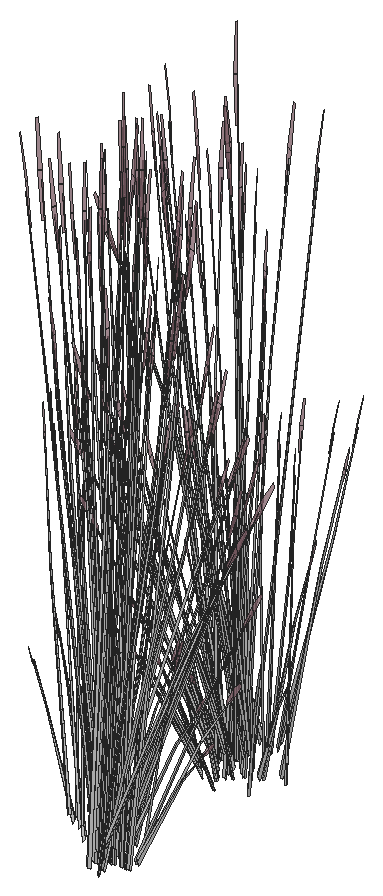
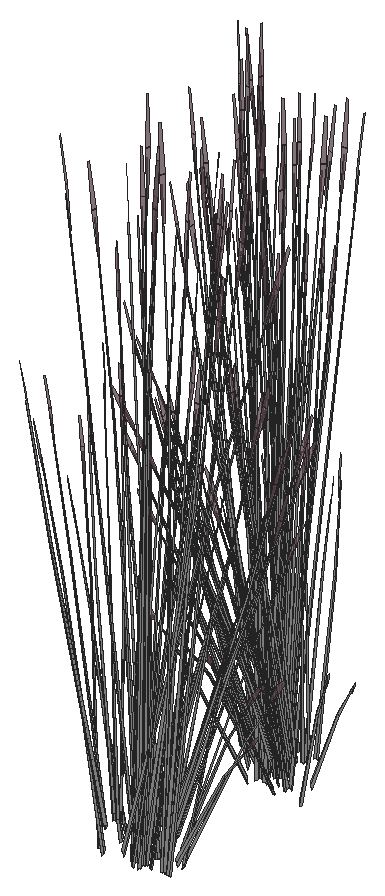
# SketchUp Ruby script. Lengths in inches.
U = 1.inch
M = Sketchup.active_model
def pt(a) = Geom::Point3d.new(a.map { |v| v * U })
def face(e, loops, mat)
  f = e.add_face(loops[0].map { |a| pt(a) })
  loops[1..].each { |l| e.add_face(l.map { |a| pt(a) }).erase! }
  f.material = f.back_material = mat if mat
  f
end
# faces: each face lists its corners as indices into pts; further lists are holes
def faces(e, pts, list, mat = nil) = list.each { |f| face(e, (f[0].is_a?(Array) ? f : [f]).map { |l| l.map { |i| pts[i] } }, mat) }
# xy, xz, yz: faces in a plane at the given z, y or x. An outline is a flat list of corners, or four numbers for a rectangle; further outlines are holes
def ring(l) = l.size == 4 ? [[l[0], l[1]], [l[2], l[1]], [l[2], l[3]], [l[0], l[3]]] : l.each_slice(2).to_a
def flat(e, list, mat, &to3) = list.each { |f| face(e, (f[0].is_a?(Array) ? f : [f]).map { |l| ring(l).map { |u, v| to3.(u, v) } }, mat) }
def xy(e, z, list, mat = nil) = flat(e, list, mat) { |x, y| [x, y, z] }
def xz(e, y, list, mat = nil) = flat(e, list, mat) { |x, z| [x, y, z] }
def yz(e, x, list, mat = nil) = flat(e, list, mat) { |y, z| [x, y, z] }
def lines(e, pts, list) = list.each { |a, b| e.add_line(pt(pts[a]), pt(pts[b])) }
# prism: a flat outline (further loops are holes) pulled along v
def prism(e, loops, v, mat = nil)
  f = face(e, loops, mat); d = Geom::Vector3d.new(v.map { |x| x * U })
  f.pushpull(f.normal.samedirection?(d) ? d.length : -d.length)
end
def box(e, o, s, mat = nil) = prism(e, [[o, [o[0] + s[0], o[1], o[2]], [o[0] + s[0], o[1] + s[1], o[2]], [o[0], o[1] + s[1], o[2]]]], [0, 0, s[2]], mat)
def at(x, y, z, deg = 0) = Geom::Transformation.translation(pt([x, y, z])) * Geom::Transformation.rotation(ORIGIN, Z_AXIS, deg.degrees)
def axes(o, x, y, z) = Geom::Transformation.new([*x, 0, *y, 0, *z, 0, *pt(o).to_a, 1])
def part(name) = M.definitions.add(name)
# library, detail: a bought-in or finely detailed component or shape, given as its bounding box
def library(name, o, s) = part(name).tap { |d| box(d.entities, o, s) }
def detail(e, o, s) = box(e.add_group.entities, o, s)
def put(e, d, t, mat = nil) = e.add_instance(d, t).tap { |i| i.material = mat if mat }
def group(e, t, mat = nil) = e.add_group.tap { |g| g.transformation = t; g.material = mat if mat }.entities
root = M.entities
M.materials.add("LightPink_Translucent").color = [144, 107, 117]
M.materials["LightPink_Translucent"].alpha = 0.75
M.materials.add("[_0053_Ivory_]").color = [200, 200, 200]
c1 = part("blade")
p = [[2.15,0.21,22],[0,0.17,0],[0.09,0.45,0],[2.18,0.31,22],[2.29,0.31,22],[0.38,0.45,0],
  [2.48,0.24,33],[2.49,0.24,33],[2.48,0.22,33]]
faces(c1.entities,p,[[0,1,2,3],[4,5,2,3],[6,3,4,7],[8,0,3,6]])
c2 = part("seeds")
p = [[0.3,-0.1,1.38],[-0.01,-0.03,1.59],[-0.01,-0.03,0.03],[0.14,-0.07,-0.07],[0.29,-0.03,3],[0.15,0.01,3.11]]
faces(c2.entities,p,[[0,1,2,3],[1,0,4,5]],"LightPink_Translucent")
c3 = part("blade with seeds")
put(c3.entities,c1,at(0,0,0))
put(c3.entities,c2,axes([2.4,0.25,30.99],[1.5799,-0.05474,1.17369],[-0.12525,1.92788,0.29478],[-0.07173,-0.02425,1.56792]))
put(root,c3,axes([645.01,152.18,129.13],[-0.65264,0.16691,0.17642],[-0.16115,-0.62115,0.35086],[0.05821,0.0905,1.60407]),"[_0053_Ivory_]")
put(root,c3,axes([645.42,153.49,130.53],[-0.25192,0.01424,1.71376],[0.16712,-0.61729,0.13857],[0.35901,0.03818,0.73262]),"[_0053_Ivory_]")
put(root,c3,axes([645.74,152.15,128.68],[0.14267,0.54795,-0.30978],[-0.56663,0.1556,0.30978],[0.11423,0.06319,1.38974]),"[_0053_Ivory_]")
put(root,c3,axes([644.6,153.375,129.03],[-0.76764,-0.13249,0.49198],[0.15622,-0.74829,0.19306],[0.11218,0.07226,1.70813]),"[_0053_Ivory_]")
put(root,c3,axes([643.99,155.22,128.86],[-0.19817,-0.54216,0],[0.56587,-0.18986,0],[0,0,1.54371]),"[_0053_Ivory_]")
put(root,c3,axes([643.61,154.71,129.27],[-0.11717,0.56122,0.1448],[-0.57245,-0.09742,-0.41347],[-0.10418,-0.05763,1.26744]),"[_0053_Ivory_]")
put(root,c3,axes([644.73,155.14,128.84],[0.63764,-0.21337,-0.19198],[0.22406,0.61462,0.00008],[0.07038,-0.02358,1.73897]),"[_0053_Ivory_]")
put(root,c3,axes([644.95,155.4,129.13],[0.17545,-0.62497,0.17642],[0.64204,0.17686,0.35086],[-0.11091,0.00304,1.60407]),"[_0053_Ivory_]")
put(root,c3,axes([644.81,153.98,128.87],[0.42396,0.40619,0],[-0.42396,0.40619,0],[0,0,1.69266]),"[_0053_Ivory_]")
put(root,c3,axes([645.95,153.81,129.13],[-0.47719,-0.45806,0.17642],[0.48088,-0.44429,0.35086],[-0.0527,0.09355,1.60407]),"[_0053_Ivory_]")
put(root,c3,axes([645.07,153.12,128.71],[0.63179,0.1031,-0.62353],[-0.13332,0.63596,-0.16365],[0.18854,0.07706,1.37633]),"[_0053_Ivory_]")
put(root,c3,axes([647.86,154.23,129.42],[-0.37526,0.10382,1.1486],[0.17664,-0.42906,0.84392],[0.19907,0.02936,0.25299]),"[_0053_Ivory_]")
put(root,c3,axes([643.85,155.47,128.85],[-0.61229,-0.28233,0],[0.29468,-0.58663,0],[0,0,1.62707]),"[_0053_Ivory_]")
put(root,c3,axes([644.36,154.71,129.12],[-0.59306,-0.50614,-0.25192],[0.49904,-0.56836,0.5513],[-0.1597,0.05921,1.68216]),"[_0053_Ivory_]")
put(root,c3,axes([642.8,155.68,129.13],[0.56842,0.31443,0.49651],[-0.33976,0.56381,0],[-0.12946,-0.07161,1.57504]),"[_0053_Ivory_]")
put(root,c3,axes([644.8,153.51,129.37],[0.29468,-0.56664,0.44739],[0.61229,0.27271,-0.21531],[0,0.13062,1.43643]),"[_0053_Ivory_]")
put(root,c3,axes([644.6875,153.83,128.95],[0,0.72727,-0.05637],[-0.75945,0,0],[0,0.02286,1.79368]),"[_0053_Ivory_]")
put(root,c3,axes([644.74,153.32,128.86],[0.36485,0.52782,-0.44739],[-0.55265,0.37168,0.21531],[0.11807,0.06531,1.43643]),"[_0053_Ivory_]")
put(root,c3,axes([647.21,155.55,130.58],[-0.11624,-0.52862,-0.03492],[0.54943,-0.12153,-0.15832],[0.11473,0.03351,0.52218]),"[_0053_Ivory_]")
put(root,c3,axes([642.47,156.01,129.03],[-0.37973,0.63014,0],[-0.6353,-0.35142,-0.51607],[-0.14469,-0.08004,1.63711]),"[_0053_Ivory_]")
put(root,c3,axes([646.35,153.82,129.13],[0,-0.62885,0.49651],[0.67951,0,0],[0,0.14322,1.57504]),"[_0053_Ivory_]")
put(root,c3,axes([644.65,154.29,129.37],[0.65953,-0.03882,0.44739],[0.05964,0.64439,-0.21531],[-0.11807,0.06531,1.43643]),"[_0053_Ivory_]")
put(root,c3,axes([645.06,153.64,129.27],[0.56587,-0.18339,0.1448],[0.19817,0.52368,-0.41347],[0,0.11525,1.26744]),"[_0053_Ivory_]")
put(root,c3,axes([644.06,154.61,128.86],[-0.65953,0.03882,-0.44739],[-0.05964,-0.64439,0.21531],[-0.11807,0.06531,1.43643]),"[_0053_Ivory_]")
put(root,c3,axes([647.16,154.91,129.24],[-0.14627,-0.15466,1.43002],[0.19032,-0.51164,-0.30754],[0.29594,0.06931,0.61141]),"[_0053_Ivory_]")
put(root,c3,axes([644.55,155.48,128.86],[0.61229,0.28233,0],[-0.29468,0.58663,0],[0,0,1.74954]),"[_0053_Ivory_]")
put(root,c3,axes([644.79,156.1,128.85],[-0.37499,-0.63235,-0.05142],[0.6353,-0.35142,0.51607],[-0.15655,0.0602,1.6363]),"[_0053_Ivory_]")
put(root,c3,axes([644.66,154.57,129.27],[0.44871,0.37783,0.1448],[-0.37428,0.42627,-0.41347],[-0.10418,0.05763,1.26744]),"[_0053_Ivory_]")
put(root,c3,axes([645.82,155.23,131.63],[0.60713,0.01514,-0.71045],[-0.04078,0.63759,0.08574],[0.25721,0.06729,1.00501]),"[_0053_Ivory_]")
put(root,c3,axes([645.13,155.74,129.13],[0.56842,-0.31443,0.49651],[0.33976,0.56381,0],[-0.12946,0.07161,1.57504]),"[_0053_Ivory_]")
put(root,c3,axes([644.32,155.24,128.94],[0.26406,0.72244,-0.06012],[-0.7545,0.25315,0],[0.00922,0.02523,1.72173]),"[_0053_Ivory_]")
put(root,c3,axes([644.62,156.02,128.68],[-0.56663,-0.1556,-0.30978],[0.14267,-0.54795,0.30978],[-0.11423,0.06319,1.38974]),"[_0053_Ivory_]")
put(root,c3,axes([646.81,153.93,129.03],[0.75945,0,0],[0,0.70283,-0.51607],[0,0.16007,1.63711]),"[_0053_Ivory_]")
put(root,c3,axes([646.51,154.29,128.85],[-0.75908,-0.00503,-0.04976],[0,-0.70283,0.49943],[-0.02386,0.16,1.58352]),"[_0053_Ivory_]")
put(root,c3,axes([644.86,153.68,129.32],[0.68399,0.30005,-0.29095],[-0.32934,0.63331,-0.50002],[0.0215,0.15549,1.59708]),"[_0053_Ivory_]")
put(root,c3,axes([640.09,156.01,129.42],[0.25312,-0.28501,1.1486],[0.09988,0.45119,0.84392],[-0.18292,0.08079,0.25299]),"[_0053_Ivory_]")
put(root,c3,axes([646.18,155.49,131.18],[0.34557,0.39372,-0.35414],[-0.39459,0.37271,0.4572],[0.20048,0.05671,0.87481]),"[_0053_Ivory_]")
put(root,c3,axes([646.35,154.39,128.68],[-0.42396,0.39235,-0.30978],[-0.42396,-0.39235,0.30978],[0,0.12637,1.38974]),"[_0053_Ivory_]")
put(root,c3,axes([644.52,154.43,129.32],[0.07077,0.71755,-0.29095],[-0.73712,0.04339,-0.50002],[-0.1298,0.09558,1.59708]),"[_0053_Ivory_]")
put(root,c3,axes([644.79,154.15,128.86],[-0.29468,0.56664,-0.44739],[-0.61229,-0.27271,0.21531],[0,0.13062,1.43643]),"[_0053_Ivory_]")
put(root,c3,axes([641.04,154.78,131.18],[-0.52868,0.08987,-0.35414],[-0.1396,-0.51376,0.4572],[-0.1515,0.13799,0.87481]),"[_0053_Ivory_]")
put(root,c3,axes([644.08,154.98,128.71],[-0.40909,0.47266,-0.62353],[-0.50819,-0.4286,-0.16365],[-0.16393,0.11791,1.37633]),"[_0053_Ivory_]")
put(root,c3,axes([644.81,155.78,128.98],[0.76036,0.2044,0.30756],[-0.19023,0.7306,-0.36492],[-0.12585,0.09144,1.64885]),"[_0053_Ivory_]")
put(root,c3,axes([644.75,156.27,128.67],[-0.56842,0.31443,-0.49651],[-0.33976,-0.56381,0],[-0.12946,0.07161,1.57504]),"[_0053_Ivory_]")
put(root,c3,axes([646.64,154.41,128.67],[0,0.62885,-0.49651],[-0.67951,0,0],[0,0.14322,1.57504]),"[_0053_Ivory_]")
put(root,c3,axes([644.94,154.48,130.53],[-0.2256,-0.10835,1.71376],[0.46687,-0.45453,0.13857],[0.29098,0.20505,0.73262]),"[_0053_Ivory_]")
put(root,c3,axes([645.78,155.71,129.42],[-0.34197,-0.18082,1.1486],[0.44156,-0.18372,0.84392],[0.1191,0.15563,0.25299]),"[_0053_Ivory_]")
put(root,c3,axes([641.96,154.28,130.53],[0.1517,-0.19322,1.71376],[0.38303,0.52154,0.13857],[-0.26271,0.23751,0.73262]),"[_0053_Ivory_]")
put(root,c3,axes([641.48,154.84,131.33],[0.15602,0.5742,-0.51099],[-0.59087,0.10045,-0.3958],[-0.16933,0.15423,0.97773]),"[_0053_Ivory_]")
put(root,c3,axes([645.27,156.17,129.03],[0.37973,0.63014,0],[-0.6353,0.35142,-0.51607],[-0.14469,0.08004,1.63711]),"[_0053_Ivory_]")
put(root,c3,axes([645.87,156.38,128.15],[0.04425,-0.09079,1.76342],[0.55709,-0.26738,-0.26939],[0.16889,0.13839,0.30037]),"[_0053_Ivory_]")
put(root,c3,axes([644.94,153.68,129.5],[-0.01659,-0.59209,1.41272],[0.75089,0.15348,0.59816],[-0.1776,0.32398,1.3335]),"[_0053_Ivory_]")
put(root,c3,axes([645.14,154.32,128.75],[0.2227,0.57576,-0.69212],[-0.64151,0.20736,-0.18165],[0.02462,0.19497,1.52773]),"[_0053_Ivory_]")
put(root,c3,axes([640.76,156.31,128.15],[0.08147,0.06283,1.76342],[0.13814,0.58211,-0.26939],[-0.18056,0.12413,0.30037]),"[_0053_Ivory_]")
put(root,c3,axes([645,155.96,131.33],[0.59932,-0.14948,-0.51099],[0.10484,0.56611,-0.3958],[0.16097,0.16223,0.97773]),"[_0053_Ivory_]")
put(root,c3,axes([645.83,156.54,129.32],[-0.38947,-0.01972,1.0506],[0.25721,-0.41888,0.58006],[0.15386,0.14882,0.8241]),"[_0053_Ivory_]")
put(root,c3,axes([641.84,154.75,130.53],[0.11309,-0.21615,1.71376],[0.47441,0.44731,0.13857],[-0.21402,0.27879,0.73262]),"[_0053_Ivory_]")
put(root,c3,axes([644.56,155.52,129.24],[0.01072,-0.20846,1.43002],[0.51218,-0.23285,-0.30754],[0.15811,0.2495,0.61141]),"[_0053_Ivory_]")
put(root,c3,axes([641.97,155.97,131.18],[-0.41095,0.33109,-0.35414],[-0.38901,-0.37805,0.4572],[-0.05919,0.19208,0.87481]),"[_0053_Ivory_]")
put(root,c3,axes([642.24,157.26,129.42],[-0.01572,-0.37392,1.1486],[0.39276,0.26669,0.84392],[-0.07724,0.17822,0.25299]),"[_0053_Ivory_]")
put(root,c3,axes([643.27,156.36,128.15],[0.09829,-0.03422,1.76342],[0.59126,0.18834,-0.26939],[0.01729,0.21228,0.30037]),"[_0053_Ivory_]")
put(root,c3,axes([642.38,155.82,131.66],[0.43478,0.42253,-0.5672],[-0.45929,0.37004,-0.43934],[-0.06615,0.21468,1.08528]),"[_0053_Ivory_]")
put(root,c3,axes([641.91,156.45,129.48],[0.55175,-0.11136,0.06507],[0.12684,0.44864,-0.86304],[-0.03498,0.22711,0.7736]),"[_0053_Ivory_]")
put(root,c3,axes([643.67,156.22,131.33],[0.59704,0.15764,-0.51099],[-0.20464,0.54049,-0.3958],[0.05475,0.21761,0.97773]),"[_0053_Ivory_]")
put(root,c3,axes([644.01,155.11,130.53],[-0.13883,-0.2019,1.71376],[0.64153,-0.16998,0.13857],[0.14499,0.31697,0.73262]),"[_0053_Ivory_]")
put(root,c3,axes([643.4,156.56,131.18],[-0.1831,0.48359,-0.35414],[-0.53419,-0.14105,0.4572],[0.04898,0.1947,0.87481]),"[_0053_Ivory_]")
put(root,c3,axes([642.25,155.62,131.99],[-0.0158,0.58168,-0.7886],[-0.66548,-0.03907,0.09517],[-0.07023,0.24643,1.11556]),"[_0053_Ivory_]")
put(root,c3,axes([642.88,155.21,130.53],[-0.01487,-0.24136,1.71376],[0.64429,0.16012,0.13857],[-0.03985,0.34396,0.73262]),"[_0053_Ivory_]")
put(root,c3,axes([643.46,156.12,131.63],[0.28988,0.51132,-0.71045],[-0.59671,0.28496,0.08574],[0.06778,0.24706,1.00501]),"[_0053_Ivory_]")
put(root,c3,axes([641.78,156.93,129.24],[0.19166,-0.0992,1.43002],[0.4732,0.29912,-0.30754],[-0.14084,0.25882,0.61141]),"[_0053_Ivory_]")
put(root,c3,axes([642.03,156.44,130.02],[0.01334,-0.32463,1.54345],[0.60018,0.17147,0.21329],[-0.052,0.34598,0.72882]),"[_0053_Ivory_]")
put(root,c3,axes([642.49,169.64,130.53],[0.13883,0.2019,1.71376],[-0.64153,0.16998,0.13857],[-0.14499,-0.31697,0.73262]),"[_0053_Ivory_]")
put(root,c3,axes([644.98,169.35,129.24],[-0.17264,0.12729,1.43002],[-0.51703,-0.22279,-0.30754],[0.09584,-0.27707,0.61141]),"[_0053_Ivory_]")
put(root,c3,axes([644.2,169.79,131.63],[-0.28988,-0.51132,-0.71045],[0.59671,-0.28496,0.08574],[-0.06778,-0.24706,1.00501]),"[_0053_Ivory_]")
put(root,c3,axes([642.3125,169.11,129.24],[-0.03678,0.20572,1.43002],[-0.53767,0.17221,-0.30754],[-0.12568,-0.26589,0.61141]),"[_0053_Ivory_]")
put(root,c3,axes([643.7,168.66,128.15],[-0.10187,0.02266,1.76342],[-0.56336,-0.25503,-0.26939],[0.00945,-0.21273,0.30037]),"[_0053_Ivory_]")
put(root,c3,axes([645.4,170.29,131.63],[0.0158,-0.58168,-0.71045],[0.66548,0.03907,0.08574],[0.07023,-0.24643,1.00501]),"[_0053_Ivory_]")
put(root,c3,axes([644.25,169.36,131.18],[0.1831,-0.48359,-0.35414],[0.53419,0.14105,0.4572],[-0.04898,-0.1947,0.87481]),"[_0053_Ivory_]")
put(root,c3,axes([644.65,170,130.53],[-0.11309,0.21615,1.71376],[-0.47441,-0.44731,0.13857],[0.21402,-0.27879,0.73262]),"[_0053_Ivory_]")
put(root,c3,axes([643.98,169.6875,131.33],[-0.59704,-0.15764,-0.51099],[0.20464,-0.54049,-0.3958],[-0.05475,-0.21761,0.97773]),"[_0053_Ivory_]")
put(root,c3,axes([644.35,168.33,129.42],[0.07791,0.3667,1.1486],[-0.43222,-0.2031,0.84392],[0.04651,-0.18776,0.25299]),"[_0053_Ivory_]")
put(root,c3,axes([645.27,170.1,131.33],[-0.43478,-0.42253,-0.51099],[0.45929,-0.37004,-0.3958],[0.06615,-0.21468,0.97773]),"[_0053_Ivory_]")
put(root,c3,axes([645.68,169.94,131.18],[0.41095,-0.33109,-0.35414],[0.38901,0.37805,0.4572],[0.05919,-0.19208,0.87481]),"[_0053_Ivory_]")
put(root,c3,axes([642.125,168.77,129.42],[0.31682,0.21887,1.1486],[-0.4614,0.13157,0.84392],[-0.09872,-0.16821,0.25299]),"[_0053_Ivory_]")
put(root,c3,axes([642.89,169.94,131.63],[-0.51789,-0.30395,-0.71045],[0.36805,-0.53263,0.08574],[-0.18764,-0.18149,1.00501]),"[_0053_Ivory_]")
put(root,c3,axes([642.71,169.53,131.18],[-0.0938,-0.50652,-0.35414],[0.53623,-0.13375,0.4572],[-0.14403,-0.14515,0.87481]),"[_0053_Ivory_]")
put(root,c3,axes([641.875,169.43,128.15],[-0.05883,0.08284,1.76342],[-0.59454,0.17861,-0.26939],[-0.14363,-0.16248,0.30037]),"[_0053_Ivory_]")
put(root,c3,axes([642.86,171.71,128.75],[-0.24943,-0.64486,-0.69835],[0.71849,-0.23224,-0.18329],[-0.02757,-0.21836,1.54149]),"[_0053_Ivory_]")
put(root,c3,axes([646.19,169.74,128.15],[-0.0909,-0.04954,1.76342],[-0.2335,-0.55347,-0.26939],[0.15752,-0.1502,0.30037]),"[_0053_Ivory_]")
put(root,c3,axes([642.65,169.95,131.33],[-0.59932,0.14948,-0.51099],[-0.10484,-0.56611,-0.3958],[-0.16097,-0.16223,0.97773]),"[_0053_Ivory_]")
put(root,c3,axes([646.1875,171.3,131.63],[0.31725,-0.49618,-0.71045],[0.55593,0.35263,0.08574],[0.18942,-0.17977,1.00501]),"[_0053_Ivory_]")
put(root,c3,axes([642.76,169.86,129.03],[-0.37973,-0.63014,0],[0.6353,-0.35142,-0.51607],[0.14469,-0.08004,1.63711]),"[_0053_Ivory_]")
put(root,c3,axes([646.17,171.07,131.33],[-0.15602,-0.5742,-0.51099],[0.59087,-0.10045,-0.3958],[0.16933,-0.15423,0.97773]),"[_0053_Ivory_]")
put(root,c3,axes([643.59,169.1,128.78],[-0.4197,0.36076,-0.03893],[-0.38456,-0.39511,-0.17649],[-0.02707,-0.11196,0.58215]),"[_0053_Ivory_]")
put(root,c3,axes([644.13,173.375,129.98],[0.52485,0.25358,1.51261],[-0.51417,0.54629,0.59816],[-0.23031,-0.32378,1.26806]),"[_0053_Ivory_]")
put(root,c3,axes([641.39,171.62,128.67],[0,-0.62885,-0.49651],[0.67951,0,0],[0,-0.14322,1.57504]),"[_0053_Ivory_]")
put(root,c3,axes([643.27,169.76,128.67],[0.56842,-0.31443,-0.49651],[0.33976,0.56381,0],[0.12946,-0.07161,1.57504]),"[_0053_Ivory_]")
put(root,c3,axes([646.65,170.85,129.24],[-0.21697,-0.01863,1.43002],[-0.22228,-0.49966,-0.30754],[0.26655,-0.14135,0.61141]),"[_0053_Ivory_]")
put(root,c3,axes([643.95,171.05,128.71],[0.40909,-0.47266,-0.62353],[0.50819,0.4286,-0.16365],[0.16393,-0.11791,1.37633]),"[_0053_Ivory_]")
put(root,c3,axes([646.9,169.93,129.42],[-0.2023,0.32011,1.1486],[-0.17388,-0.43009,0.84392],[0.16708,-0.10777,0.25299]),"[_0053_Ivory_]")
put(root,c3,axes([646.61,171.13,131.18],[0.52868,-0.08987,-0.35414],[0.1396,0.51376,0.4572],[0.1515,-0.13799,0.87481]),"[_0053_Ivory_]")
put(root,c3,axes([643.24,171.88,128.86],[0.29468,-0.56664,-0.44739],[0.61229,0.27271,0.21531],[0,-0.13062,1.43643]),"[_0053_Ivory_]")
put(root,c3,axes([641.47,170.42,131.18],[-0.34557,-0.39372,-0.35414],[0.39459,-0.37271,0.4572],[-0.20048,-0.05671,0.87481]),"[_0053_Ivory_]")
put(root,c3,axes([643.5,171.6,129.32],[-0.07077,-0.71755,-0.29095],[0.73712,-0.04339,-0.50002],[0.1298,-0.09558,1.59708]),"[_0053_Ivory_]")
put(root,c3,axes([641.68,171.63,128.68],[0.42396,-0.39235,-0.30978],[0.42396,0.39235,0.30978],[0,-0.12637,1.38974]),"[_0053_Ivory_]")
put(root,c3,axes([641.51,169.75,128.78],[-0.1752,0.51349,-0.03893],[-0.53924,-0.15795,-0.17649],[-0.08187,-0.08399,0.58215]),"[_0053_Ivory_]")
put(root,c3,axes([643.16,172.35,129.32],[-0.68399,-0.30005,-0.29095],[0.32934,-0.63331,-0.50002],[-0.0215,-0.15549,1.59708]),"[_0053_Ivory_]")
put(root,c3,axes([641.22,172.1,129.03],[-0.75945,0,0],[0,-0.70283,-0.51607],[0,-0.16007,1.63711]),"[_0053_Ivory_]")
put(root,c3,axes([643.41,170.01,128.68],[0.56663,0.1556,-0.30978],[-0.14267,0.54795,0.30978],[0.11423,-0.06319,1.38974]),"[_0053_Ivory_]")
put(root,c3,axes([641.8,171.91,128.98],[-0.56493,0.5287,0.30756],[-0.56528,-0.52313,-0.36492],[-0.01973,-0.15014,1.64885]),"[_0053_Ivory_]")
put(root,c3,axes([643.6,172.16,129.09],[0.68433,0.30479,0.24065],[-0.32934,0.63331,0.50002],[0,-0.14599,1.60543]),"[_0053_Ivory_]")
put(root,c3,axes([643.33,173.01,129.09],[0.16098,-0.74515,-0.23429],[0.76326,0.12989,0.51271],[-0.13337,-0.1029,1.5644]),"[_0053_Ivory_]")
put(root,c3,axes([640.64,171.37,129.42],[0.38775,-0.045,1.1486],[-0.24596,0.39648,0.84392],[-0.19161,-0.05948,0.25299]),"[_0053_Ivory_]")
put(root,c3,axes([643.38,171.73,129.37],[-0.65953,0.03882,0.44739],[-0.05964,-0.64439,-0.21531],[0.11807,-0.06531,1.43643]),"[_0053_Ivory_]")
put(root,c3,axes([641.68,172.2,129.13],[0,0.62885,0.49651],[-0.67951,0,0],[0,-0.14322,1.57504]),"[_0053_Ivory_]")
put(root,c3,axes([646.45,172.34,131.33],[0.16454,-0.57202,-0.51099],[0.56413,0.19607,-0.3958],[0.22713,-0.05245,0.97773]),"[_0053_Ivory_]")
put(root,c3,axes([645.55,170.02,129.03],[0.37973,-0.63014,0],[0.6353,0.35142,-0.51607],[0.14469,0.08004,1.63711]),"[_0053_Ivory_]")
put(root,c3,axes([643.28,172.71,128.86],[-0.36485,-0.52782,-0.44739],[0.55265,-0.37168,0.21531],[-0.11807,-0.06531,1.43643]),"[_0053_Ivory_]")
put(root,c3,axes([643.36,171.97,129.01],[0.26406,0.70318,0.45755],[-0.7545,0.24452,0.17955],[0.00922,-0.12921,1.58856]),"[_0053_Ivory_]")
put(root,c3,axes([647.05,172.51,128.64],[-0.39118,0.07547,1.41583],[-0.06226,-0.6007,0.08104],[0.27398,-0.09092,0.80566]),"[_0053_Ivory_]")
put(root,c3,axes([647.76,171.97,128.91],[-0.37654,-0.40212,-0.06488],[0.4124,-0.36845,-0.29416],[0.11685,-0.02594,0.97024]),"[_0053_Ivory_]")
put(root,c3,axes([643.22,172.52,129.37],[-0.29468,0.56664,0.44739],[-0.61229,-0.27271,-0.21531],[0,-0.13062,1.43643]),"[_0053_Ivory_]")
put(root,c3,axes([644.31,172.03,128.86],[0,-0.72763,0],[0.75945,0,0],[0,0,1.79456]),"[_0053_Ivory_]")
put(root,c3,axes([645.23,170.34,129.13],[-0.56842,-0.31443,0.49651],[0.33976,-0.56381,0],[0.12946,0.07161,1.57504]),"[_0053_Ivory_]")
put(root,c3,axes([646.34,172.55,131.63],[0.53369,-0.27773,-0.71045],[0.29743,0.5717,0.08574],[0.25786,-0.06494,1.00501]),"[_0053_Ivory_]")
